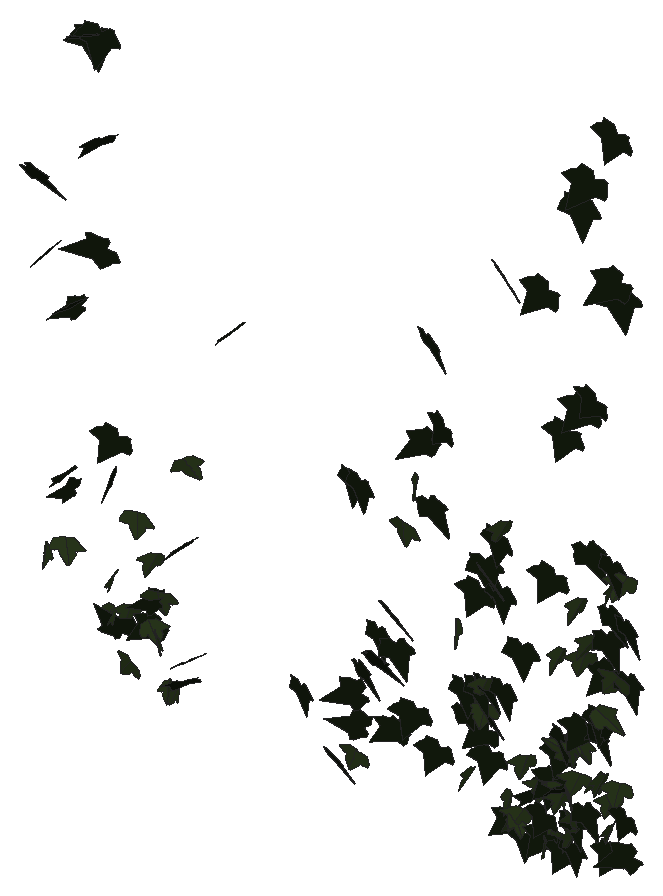
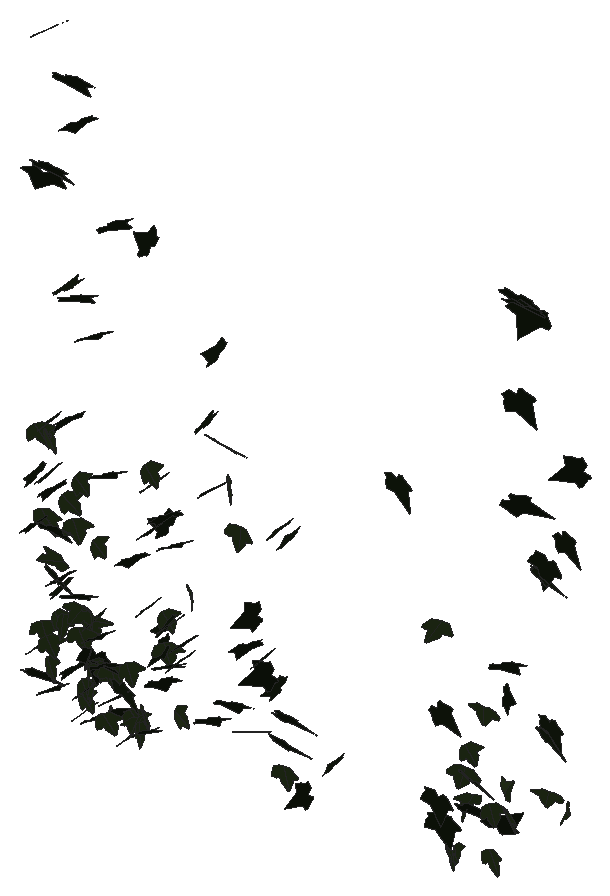
# SketchUp Ruby script. Lengths in inches.
U = 1.inch
M = Sketchup.active_model
def pt(a) = Geom::Point3d.new(a.map { |v| v * U })
def face(e, loops, mat)
  f = e.add_face(loops[0].map { |a| pt(a) })
  loops[1..].each { |l| e.add_face(l.map { |a| pt(a) }).erase! }
  f.material = f.back_material = mat if mat
  f
end
# faces: each face lists its corners as indices into pts; further lists are holes
def faces(e, pts, list, mat = nil) = list.each { |f| face(e, (f[0].is_a?(Array) ? f : [f]).map { |l| l.map { |i| pts[i] } }, mat) }
# xy, xz, yz: faces in a plane at the given z, y or x. An outline is a flat list of corners, or four numbers for a rectangle; further outlines are holes
def ring(l) = l.size == 4 ? [[l[0], l[1]], [l[2], l[1]], [l[2], l[3]], [l[0], l[3]]] : l.each_slice(2).to_a
def flat(e, list, mat, &to3) = list.each { |f| face(e, (f[0].is_a?(Array) ? f : [f]).map { |l| ring(l).map { |u, v| to3.(u, v) } }, mat) }
def xy(e, z, list, mat = nil) = flat(e, list, mat) { |x, y| [x, y, z] }
def xz(e, y, list, mat = nil) = flat(e, list, mat) { |x, z| [x, y, z] }
def yz(e, x, list, mat = nil) = flat(e, list, mat) { |y, z| [x, y, z] }
def lines(e, pts, list) = list.each { |a, b| e.add_line(pt(pts[a]), pt(pts[b])) }
# prism: a flat outline (further loops are holes) pulled along v
def prism(e, loops, v, mat = nil)
  f = face(e, loops, mat); d = Geom::Vector3d.new(v.map { |x| x * U })
  f.pushpull(f.normal.samedirection?(d) ? d.length : -d.length)
end
def box(e, o, s, mat = nil) = prism(e, [[o, [o[0] + s[0], o[1], o[2]], [o[0] + s[0], o[1] + s[1], o[2]], [o[0], o[1] + s[1], o[2]]]], [0, 0, s[2]], mat)
def at(x, y, z, deg = 0) = Geom::Transformation.translation(pt([x, y, z])) * Geom::Transformation.rotation(ORIGIN, Z_AXIS, deg.degrees)
def axes(o, x, y, z) = Geom::Transformation.new([*x, 0, *y, 0, *z, 0, *pt(o).to_a, 1])
def part(name) = M.definitions.add(name)
# library, detail: a bought-in or finely detailed component or shape, given as its bounding box
def library(name, o, s) = part(name).tap { |d| box(d.entities, o, s) }
def detail(e, o, s) = box(e.add_group.entities, o, s)
def put(e, d, t, mat = nil) = e.add_instance(d, t).tap { |i| i.material = mat if mat }
def group(e, t, mat = nil) = e.add_group.tap { |g| g.transformation = t; g.material = mat if mat }.entities
root = M.entities
M.materials.add("1026 AP 7946 SUNNY SIDE UP").color = [254, 231, 186]
M.materials.add("efeu1").color = [18, 25, 13]
M.materials.add("efeu2").color = [43, 57, 29]
c1 = part("ivyleaf_9")
p = [[1.54,2.16,1.25],[1.36,2.04,1.19],[-0.21,0.99,0.68],[-0.71,1.11,0.82],[-0.85,0.86,0.67],[-0.8,0.17,0.21],
  [-0.9,-0.01,0.1],[-0.67,-0.16,-0.02],[-0.08,-0.08,-0.05],[-0.03,-0.6,-0.4],[0.65,-0.88,-0.66],[0.83,-0.6,-0.49],
  [1.29,-0.42,-0.43],[1.8125,-0.07,-0.26],[1.21,0.44,0.15]]
faces(c1.entities,p,[[0,1,2,3,4,5,6,7,8,9,10,11,12,13,14]],"efeu1")
c2 = part("ivyleaf_10")
p = [[0,0.5,-0.03],[-0.0625,2.02,-0.43],[-0.19,2.01,-0.46],[-0.54,1.05,-0.29],[-0.52,0.625,-0.18],[-0.83,0.76,-0.28],
  [-1.16,0.64,-0.33],[-1.15,0.33,-0.24],[-0.77,-0.39,0.02],[-0.3,-0.51,0.16],[0.04,-0.48,0.23],[-0.02,2.01,-0.4375],
  [-0.06,2.01,-0.43],[0.04,-0.49,0.23],[0.67,-0.49,0.14],[1.38,0.36,-0.2],[1.375,0.51,-0.24],[0.81,0.65,-0.19],
  [0.62,0.59,-0.15],[0.6,1.09,-0.28],[0.5,1.23,-0.31]]
faces(c2.entities,p,[[0,1,2,3,4,5,6,7,8,9,10],[11,12,0,13,14,15,16,17,18,19,20]],"efeu2")
put(root,c1,axes([92.76,212.33,309.97],[0.61577,-0.10114,0.08621],[0.11486,-0.06042,-0.40182],[0.18865,0.36692,-0.03675]),"1026 AP 7946 SUNNY SIDE UP")
put(root,c1,axes([93.45,212.58,306.92],[-0.2298,0.32016,-0.13975],[0.08656,-0.1247,-0.37388],[-0.58325,-0.14465,-0.00043]),"1026 AP 7946 SUNNY SIDE UP")
put(root,c2,axes([93.38,212.5,295.07],[-0.02793,0.21923,-0.27285],[-0.01306,-0.2582,-0.23822],[-0.57422,-0.00479,0.01869]),"1026 AP 7946 SUNNY SIDE UP")
put(root,c1,axes([94.39,212.21,298.42],[-0.11098,0.34417,0.06318],[-0.03773,0.05125,-0.37411],[-0.59033,-0.06798,0.01203]),"1026 AP 7946 SUNNY SIDE UP")
put(root,c2,axes([94.16,212.53,295.5625],[0.52881,0.11571,0.0689],[0.11671,-0.00528,-0.35454],[-0.19063,0.31775,-0.02595]),"1026 AP 7946 SUNNY SIDE UP")
put(root,c1,axes([94.67,212.66,305.0625],[-0.51376,0.19612,-0.06721],[0.01225,-0.10575,-0.37708],[-0.3507,-0.291,0.08529]),"1026 AP 7946 SUNNY SIDE UP")
put(root,c1,axes([94.69,212.27,297.96],[-0.38076,0.27164,0.01445],[-0.03395,-0.00362,-0.37671],[-0.46018,-0.22449,0.01583]),"1026 AP 7946 SUNNY SIDE UP")
put(root,c1,axes([94.6,212.12,305.27],[0.14247,0.35425,0.11205],[0.00975,0.10134,-0.3879],[-0.6248,0.08236,0.0195]),"1026 AP 7946 SUNNY SIDE UP")
put(root,c1,axes([95.09,212.29,316.06],[0.47035,0.31068,0.05928],[-0.02815,0.08266,-0.43872],[-0.5338,0.26939,0.07537]),"1026 AP 7946 SUNNY SIDE UP")
put(root,c1,axes([95.8,212.66,307.74],[-0.10303,-0.08129,-0.39977],[-0.38932,-0.29335,0.10448],[-0.51672,0.23723,0.00098]),"1026 AP 7946 SUNNY SIDE UP")
put(root,c1,axes([95.82,212.41,312.1875],[-0.07673,0.3426,-0.20544],[-0.01788,-0.19862,-0.37118],[-0.67009,-0.03393,0.03343]),"1026 AP 7946 SUNNY SIDE UP")
put(root,c1,axes([95.49,212.48,316.25],[-0.40695,-0.24543,-0.24571],[0.43304,0.04505,-0.34098],[0.36556,-0.32658,0.13039]),"1026 AP 7946 SUNNY SIDE UP")
put(root,c1,axes([95.88,212.35,316.48],[-0.54501,-0.14123,-0.22991],[0.36523,0.03495,-0.37167],[0.2339,-0.38365,0.04465]),"1026 AP 7946 SUNNY SIDE UP")
put(root,c1,axes([96.36,212.66,300.47],[-0.43398,-0.25244,0.05353],[-0.03118,-0.05703,-0.38432],[0.43686,-0.25484,0.02575]),"1026 AP 7946 SUNNY SIDE UP")
put(root,c2,axes([96.3125,212.5,294.95],[-0.13702,-0.0091,-0.36236],[-0.03469,-0.34708,0.01037],[-0.57353,0.02317,0.08594]),"1026 AP 7946 SUNNY SIDE UP")
put(root,c1,axes([96.3125,212.52,299.07],[-0.18552,0.03168,-0.36972],[0.4272,-0.24251,-0.11233],[-0.40607,-0.2696,0.05073]),"1026 AP 7946 SUNNY SIDE UP")
put(root,c2,axes([96.43,212.23,293.77],[0.36982,-0.24987,-0.03818],[-0.05471,0.01486,-0.35436],[0.4242,0.21975,-0.01241]),"1026 AP 7946 SUNNY SIDE UP")
put(root,c1,axes([96.85,212.26,293.11],[0.19309,0.02805,0.35312],[-0.55423,0.06471,0.11568],[-0.08889,-0.3425,0.04579]),"1026 AP 7946 SUNNY SIDE UP")
put(root,c2,axes([97.13,212.41,291.84],[-0.44163,0.1062,0.2101],[-0.32935,0.03695,-0.29834],[-0.18291,-0.32294,0.0299]),"1026 AP 7946 SUNNY SIDE UP")
put(root,c2,axes([96.99,212.56,293.95],[-0.27729,-0.29083,0.06551],[0.01248,-0.07802,-0.35511],[0.50572,-0.15754,0.04469]),"1026 AP 7946 SUNNY SIDE UP")
put(root,c2,axes([97.54,212.21,297.9],[0.57977,0.00723,0.05775],[0.09081,0.01514,-0.36521],[-0.01612,0.34542,0.01963]),"1026 AP 7946 SUNNY SIDE UP")
put(root,c1,axes([98.17,212.6,293.65],[-0.544,-0.05543,0.0581],[-0.08436,-0.0344,-0.34762],[0.10224,-0.32332,0.02233]),"1026 AP 7946 SUNNY SIDE UP")
put(root,c2,axes([98,212.68,296.24],[-0.19952,-0.30194,0.13893],[-0.00662,-0.14065,-0.34565],[0.56052,-0.10914,0.04537]),"1026 AP 7946 SUNNY SIDE UP")
put(root,c1,axes([98.43,212.28,294.84],[-0.45298,0.21964,0.03461],[-0.0944,-0.02605,-0.36872],[-0.33608,-0.28872,0.05692]),"1026 AP 7946 SUNNY SIDE UP")
put(root,c2,axes([98.22,212.18,293.85],[0.28342,0.28049,0.09923],[0.04661,0.08707,-0.34757],[-0.49737,0.16799,0.02397]),"1026 AP 7946 SUNNY SIDE UP")
put(root,c2,axes([98.44,212.39,295.01],[-0.55179,-0.10051,-0.04825],[0.08139,-0.00722,-0.36366],[0.16735,-0.3279,0.01778]),"1026 AP 7946 SUNNY SIDE UP")
put(root,c2,axes([98.48,212.21,293.48],[-0.29828,0.28417,0.04966],[-0.08846,0.01768,-0.3555],[-0.47971,-0.17996,0.03468]),"1026 AP 7946 SUNNY SIDE UP")
put(root,c2,axes([98.71,212.51,291.54],[0.00491,-0.31439,0.09799],[0.17001,-0.09024,-0.32211],[0.53129,0.03178,0.10217]),"1026 AP 7946 SUNNY SIDE UP")
put(root,c2,axes([98.96,212.58,291.42],[0.3772,-0.23837,-0.04113],[-0.00122,0.04737,-0.34657],[0.40905,0.21995,0.03689]),"1026 AP 7946 SUNNY SIDE UP")
put(root,c1,axes([99.5,212.53,297.37],[-0.24023,0.28037,-0.20072],[0.05362,-0.20157,-0.3249],[-0.53561,-0.14593,0.0575]),"1026 AP 7946 SUNNY SIDE UP")
put(root,c1,axes([99.75,211.99,292.24],[0.1229,0.34201,-0.07529],[-0.10599,-0.06253,-0.37172],[-0.58476,0.08321,0.05155]),"1026 AP 7946 SUNNY SIDE UP")
put(root,c1,axes([99.99,211.99,293.14],[0.09011,0.35225,0.06284],[-0.05127,0.05895,-0.37835],[-0.6028,0.04764,0.04157]),"1026 AP 7946 SUNNY SIDE UP")
put(root,c2,axes([99.73,212.27,300.82],[-0.35864,-0.2511,-0.18487],[0.25136,0.09271,-0.34517],[0.4136,-0.27408,0.04947]),"1026 AP 7946 SUNNY SIDE UP")
put(root,c1,axes([101.59,212.46,306.54],[-0.14057,0.39503,-0.00121],[-0.01341,-0.00543,-0.41716],[-0.62102,-0.0893,0.00928]),"1026 AP 7946 SUNNY SIDE UP")
put(root,c1,axes([104.39,212.8,293.33],[0.08514,-0.33489,0.13186],[0.00493,-0.13092,-0.34982],[0.56478,0.05163,-0.01683]),"1026 AP 7946 SUNNY SIDE UP")
put(root,c1,axes([105.95,212.45,291.38],[0.52028,-0.1702,-0.03005],[-0.06115,-0.01416,-0.38214],[0.26429,0.33178,-0.02927]),"1026 AP 7946 SUNNY SIDE UP")
put(root,c1,axes([106.58,212.85,302.33],[0.03148,-0.34089,0.19903],[0.00021,-0.19538,-0.35278],[0.61761,0.01744,-0.01002]),"1026 AP 7946 SUNNY SIDE UP")
put(root,c1,axes([107.32,212.34,294.28],[-0.56788,0.06211,0.12333],[-0.19615,-0.02638,-0.37484],[-0.07932,-0.37945,0.04396]),"1026 AP 7946 SUNNY SIDE UP")
put(root,c2,axes([107.23,212.29,291.88],[-0.52801,0.04641,0.11954],[-0.19129,-0.04843,-0.34377],[-0.04332,-0.35188,0.06095]),"1026 AP 7946 SUNNY SIDE UP")
put(root,c1,axes([107.53,212.26,293.06],[-0.38427,0.1589,0.22422],[-0.34435,0.05207,-0.2934],[-0.24496,-0.32247,0.06071]),"1026 AP 7946 SUNNY SIDE UP")
put(root,c1,axes([107.15,212.64,302.49],[0.02786,-0.37071,0.13348],[0.00817,-0.13158,-0.38311],[0.61854,0.01843,-0.00095]),"1026 AP 7946 SUNNY SIDE UP")
put(root,c1,axes([107.41,212.29,295.43],[0.33607,-0.32348,0.0119],[-0.01669,-0.02304,-0.39893],[0.5088,0.2129,-0.02095]),"1026 AP 7946 SUNNY SIDE UP")
put(root,c1,axes([107.81,212.81,296.75],[0.06498,-0.36544,0.07076],[-0.0077,-0.07172,-0.37907],[0.58525,0.03963,-0.01285]),"1026 AP 7946 SUNNY SIDE UP")
put(root,c1,axes([107.82,212.41,295.88],[0.58312,-0.09763,0.07354],[0.09192,-0.05887,-0.3931],[0.16707,0.37314,-0.04039]),"1026 AP 7946 SUNNY SIDE UP")
put(root,c1,axes([108.78,212.71,293.22],[-0.47428,-0.14407,0.14753],[-0.06989,-0.2046,-0.30792],[0.31261,-0.26432,0.155]),"1026 AP 7946 SUNNY SIDE UP")
put(root,c1,axes([108.55,212.28,298.15],[0.53786,-0.20306,0.00164],[-0.02065,-0.02749,-0.40877],[0.31865,0.34097,-0.02926]),"1026 AP 7946 SUNNY SIDE UP")
put(root,c1,axes([108.94,212.36,296.77],[-0.03467,-0.37319,-0.13431],[0.01555,0.12789,-0.38437],[0.62029,-0.02406,0.00213]),"1026 AP 7946 SUNNY SIDE UP")
put(root,c2,axes([109.29,212.4,301.58],[-0.58905,0.10382,0.03928],[-0.07359,-0.02909,-0.39848],[-0.15722,-0.37537,0.03937]),"1026 AP 7946 SUNNY SIDE UP")
put(root,c1,axes([109.49,212.73,294.22],[-0.43258,-0.24305,-0.05714],[0.13844,-0.01956,-0.37091],[0.36623,-0.27969,0.07272]),"1026 AP 7946 SUNNY SIDE UP")
put(root,c2,axes([109.79,212.39,303.51],[0.27299,-0.35416,-0.05085],[0.04921,0.06751,-0.40162],[0.55968,0.16681,0.06012]),"1026 AP 7946 SUNNY SIDE UP")
put(root,c1,axes([110.26,212.58,305.25],[-0.62794,0.01764,-0.04299],[0.05227,-0.13862,-0.38795],[-0.04861,-0.37685,0.13819]),"1026 AP 7946 SUNNY SIDE UP")
put(root,c1,axes([110.05,212.73,309.19],[0.28418,-0.35183,0.13106],[0.05181,-0.12799,-0.40723],[0.58707,0.1816,-0.02751]),"1026 AP 7946 SUNNY SIDE UP")
put(root,c1,axes([110.58,212.69,293.1],[-0.34561,-0.2899,0.04054],[0.02481,-0.06291,-0.37156],[0.4597,-0.21455,0.05053]),"1026 AP 7946 SUNNY SIDE UP")
put(root,c1,axes([110.52,212.26,303.02],[0.14494,-0.37106,-0.10672],[0.03381,0.10916,-0.39043],[0.60394,0.08294,0.04747]),"1026 AP 7946 SUNNY SIDE UP")
put(root,c1,axes([110.7,212.81,305.83],[-0.1396,-0.2355,0.32488],[-0.04872,-0.31945,-0.25553],[0.61864,-0.0783,0.05319]),"1026 AP 7946 SUNNY SIDE UP")
put(root,c2,axes([111.375,212.71,298.25],[-0.29683,0.24921,-0.23039],[0.01618,-0.25376,-0.29986],[-0.52775,-0.14795,0.12039]),"1026 AP 7946 SUNNY SIDE UP")
put(root,c1,axes([111.76,212.68,295.98],[-0.01895,-0.37074,0.06366],[-0.00045,-0.06393,-0.38251],[0.59155,-0.01192,0.00175]),"1026 AP 7946 SUNNY SIDE UP")
put(root,c2,axes([112.07,212.57,292.76],[0.09882,-0.30776,0.18989],[0.03267,-0.18547,-0.32434],[0.56455,0.0646,-0.01447]),"1026 AP 7946 SUNNY SIDE UP")
put(root,c1,axes([111.87,212.46,295.23],[0.21872,-0.31701,-0.14947],[-0.05198,0.14158,-0.35491],[0.54455,0.14084,0.02616]),"1026 AP 7946 SUNNY SIDE UP")
put(root,c1,axes([112.37,212.72,300.01],[-0.28977,-0.3244,0.11851],[0.00763,-0.13495,-0.37877],[0.54213,-0.17149,0.06867]),"1026 AP 7946 SUNNY SIDE UP")
put(root,c2,axes([112.6875,212.61,295.4375],[-0.42174,-0.24526,0.08988],[0.01028,-0.13343,-0.36077],[0.40994,-0.24898,0.10151]),"1026 AP 7946 SUNNY SIDE UP")
put(root,c1,axes([112.75,212.65,294.61],[-0.39792,-0.22093,0.16301],[-0.07115,-0.18057,-0.3327],[0.4225,-0.23848,0.0975]),"1026 AP 7946 SUNNY SIDE UP")
put(root,c1,axes([112.52,212.39,296.49],[0.07628,-0.37578,-0.00629],[0.00136,0.00411,-0.39032],[0.59091,0.0485,0.00171]),"1026 AP 7946 SUNNY SIDE UP")
put(root,c1,axes([112.61,212.72,301.21],[-0.07166,-0.38594,-0.07628],[0.02447,0.0705,-0.39987],[0.61679,-0.04764,0.007]),"1026 AP 7946 SUNNY SIDE UP")
put(root,c2,axes([112.88,212.36,296.64],[-0.14948,-0.33316,0.15162],[0.0167,-0.1565,-0.35427],[0.57367,-0.08226,0.04982]),"1026 AP 7946 SUNNY SIDE UP")
put(root,c1,axes([112.57,212.65,296.49],[0.26184,-0.33798,0.03074],[0.00159,-0.03488,-0.38807],[0.53378,0.1659,-0.01392]),"1026 AP 7946 SUNNY SIDE UP")
put(root,c1,axes([112.52,212.72,300.82],[0.27578,-0.28479,0.21287],[0.14109,-0.18891,-0.34509],[0.53651,0.19606,-0.01867]),"1026 AP 7946 SUNNY SIDE UP")
put(root,c1,axes([112.72,212.53,295.49],[0.4477,-0.22274,-0.16021],[-0.21489,0.07514,-0.37122],[0.36786,0.31498,-0.02187]),"1026 AP 7946 SUNNY SIDE UP")
put(root,c1,axes([113.05,212.5,293.81],[-0.27158,-0.32542,-0.00198],[0.00749,-0.00244,-0.37951],[0.51164,-0.1727,0.0045]),"1026 AP 7946 SUNNY SIDE UP")
put(root,c1,axes([113.22,212.7,302.38],[-0.07425,-0.36005,0.16836],[0.00465,-0.16696,-0.37436],[0.62305,-0.04166,0.02286]),"1026 AP 7946 SUNNY SIDE UP")
put(root,c2,axes([113.45,212.69,302.93],[-0.08907,-0.37004,0.14562],[-0.00175,-0.14476,-0.38599],[0.62405,-0.05322,0.01971]),"1026 AP 7946 SUNNY SIDE UP")
put(root,c1,axes([113.33,212.73,300.34],[-0.02505,-0.38348,0.0777],[-0.00979,-0.0774,-0.39584],[0.61513,-0.01685,-0.00313]),"1026 AP 7946 SUNNY SIDE UP")
put(root,c1,axes([113.28,212.84,312.76],[0.19804,-0.27752,0.30493],[0.1609,-0.27988,-0.31516],[0.61924,0.16148,-0.01563]),"1026 AP 7946 SUNNY SIDE UP")
put(root,c2,axes([113.67,212.68,292.3],[0.33778,-0.28088,0.05386],[0.06429,-0.03652,-0.36435],[0.44508,0.21844,0.01176]),"1026 AP 7946 SUNNY SIDE UP")
put(root,c1,axes([113.875,212.74,291.37],[-0.35189,-0.19692,0.20702],[-0.13198,-0.19978,-0.2975],[0.42358,-0.22584,0.07929]),"1026 AP 7946 SUNNY SIDE UP")
put(root,c1,axes([113.6875,212.375,296.75],[0.05324,-0.37034,0.06676],[-0.00059,-0.06721,-0.38345],[0.59174,0.03325,-0.00639]),"1026 AP 7946 SUNNY SIDE UP")
put(root,c2,axes([113.95,212.56,291.51],[0.00925,-0.35273,-0.08524],[0.03487,0.08095,-0.36219],[0.56791,0.00077,0.02363]),"1026 AP 7946 SUNNY SIDE UP")
put(root,c2,axes([114.33,212.52,291.92],[-0.31828,-0.25071,0.17213],[-0.06358,-0.17853,-0.32472],[0.47071,-0.19364,0.07253]),"1026 AP 7946 SUNNY SIDE UP")
put(root,c2,axes([114.18,212.48,291.75],[0.17444,0.34119,0.01481],[0.03131,0.00659,-0.36916],[-0.53593,0.11144,-0.01675]),"1026 AP 7946 SUNNY SIDE UP")
put(root,c2,axes([114.4,212.7,293.99],[-0.23901,-0.32785,0.07921],[0.02709,-0.09382,-0.36868],[0.52948,-0.14319,0.05462]),"1026 AP 7946 SUNNY SIDE UP")
put(root,c1,axes([114.36,212.71,290.99],[-0.0436,-0.33417,0.11668],[0.01322,-0.1161,-0.34568],[0.55562,-0.02346,0.01738]),"1026 AP 7946 SUNNY SIDE UP")
put(root,c1,axes([114.5,212.41,298.6],[-0.11185,-0.37995,-0.02259],[0.00906,0.01904,-0.3981],[0.59817,-0.07133,0.00181]),"1026 AP 7946 SUNNY SIDE UP")
put(root,c1,axes([114.98,212.41,292.89],[-0.2038,0.33206,0.06533],[-0.10594,0.03915,-0.36367],[-0.52034,-0.13803,0.04846]),"1026 AP 7946 SUNNY SIDE UP")
put(root,c1,axes([115.3,212.76,312.88],[-0.36738,-0.30189,0.19767],[-0.15253,-0.16924,-0.39348],[0.54289,-0.25184,0.02321]),"1026 AP 7946 SUNNY SIDE UP")
put(root,c2,axes([115.4,212.47,293.44],[-0.46875,-0.19675,0.07023],[-0.06186,-0.06566,-0.36682],[0.32211,-0.29893,0.03176]),"1026 AP 7946 SUNNY SIDE UP")
put(root,c2,axes([115.5,212.7,291.43],[-0.31805,-0.25002,0.16116],[-0.074,-0.1616,-0.32674],[0.45901,-0.19929,0.059]),"1026 AP 7946 SUNNY SIDE UP")
put(root,c1,axes([115.4,212.5625,292.2],[-0.20451,-0.29488,0.17573],[-0.03763,-0.176,-0.33004],[0.53567,-0.12494,0.04391]),"1026 AP 7946 SUNNY SIDE UP")
put(root,c1,axes([115.55,212.42,291.53],[-0.32331,-0.26693,0.1284],[-0.08921,-0.11514,-0.34693],[0.45559,-0.21198,0.02319]),"1026 AP 7946 SUNNY SIDE UP")
put(root,c1,axes([115.74,212.75,293.64],[-0.40872,-0.22551,0.12154],[-0.07799,-0.12234,-0.3504],[0.39347,-0.2585,0.0568]),"1026 AP 7946 SUNNY SIDE UP")
put(root,c2,axes([115.7,212.1,291.36],[0.22946,-0.30539,-0.11619],[0.02244,0.12764,-0.34154],[0.51047,0.13166,0.06724]),"1026 AP 7946 SUNNY SIDE UP")
put(root,c2,axes([115.63,212.46,293.45],[-0.46856,-0.1327,-0.17327],[0.27078,0.02089,-0.33267],[0.19883,-0.34117,0.04473]),"1026 AP 7946 SUNNY SIDE UP")
put(root,c1,axes([115.77,212.5625,301.82],[-0.35199,-0.30882,0.10792],[0.00094,-0.12951,-0.3863],[0.51367,-0.21138,0.07466]),"1026 AP 7946 SUNNY SIDE UP")
put(root,c1,axes([115.71,212.65,293.63],[-0.43445,-0.19272,-0.1517],[0.29173,-0.02651,-0.32547],[0.244,-0.31145,0.11903]),"1026 AP 7946 SUNNY SIDE UP")
put(root,c2,axes([115.97,212.66,298.78],[-0.02909,-0.32138,0.21826],[0.07551,-0.21419,-0.32883],[0.60214,0.01134,0.05178]),"1026 AP 7946 SUNNY SIDE UP")
put(root,c1,axes([115.95,212.77,294.83],[-0.19694,-0.33442,0.105],[-0.00241,-0.10974,-0.3667],[0.5506,-0.1201,0.03595]),"1026 AP 7946 SUNNY SIDE UP")
put(root,c2,axes([116.23,212.42,293.37],[-0.1578,-0.33565,0.11967],[0.03324,-0.12808,-0.35735],[0.55849,-0.08721,0.05508]),"1026 AP 7946 SUNNY SIDE UP")
put(root,c1,axes([116.04,212.74,295.48],[0.04424,-0.34351,0.14383],[-0.00079,-0.14201,-0.35571],[0.5842,0.02582,-0.01137]),"1026 AP 7946 SUNNY SIDE UP")
put(root,c1,axes([116.34,212.24,293.67],[0.15539,0.34604,-0.05455],[-0.01018,-0.05525,-0.37096],[-0.55083,0.09864,-0.00853]),"1026 AP 7946 SUNNY SIDE UP")
put(root,c2,axes([116.64,212.42,295.14],[0.18628,0.09215,0.36401],[-0.52394,-0.12334,0.14773],[0.23292,-0.35114,0.04119]),"1026 AP 7946 SUNNY SIDE UP")
put(root,c1,axes([116.24,212.6,291.1],[-0.24012,-0.29566,0.14021],[-0.02875,-0.14414,-0.34036],[0.5121,-0.14673,0.04664]),"1026 AP 7946 SUNNY SIDE UP")
put(root,c1,axes([116.32,212.67,307.67],[-0.29672,-0.35246,0.11772],[0.00962,-0.13337,-0.40706],[0.58351,-0.17703,0.06657]),"1026 AP 7946 SUNNY SIDE UP")
put(root,c2,axes([116.37,212.6,292.49],[-0.37598,0.26177,-0.09683],[0.06818,-0.08932,-0.36469],[-0.4328,-0.24148,0.02666]),"1026 AP 7946 SUNNY SIDE UP")
put(root,c2,axes([116.57,212.66,292.49],[-0.09108,-0.35324,0.05346],[-0.00381,-0.05421,-0.36902],[0.56185,-0.05763,0.00616]),"1026 AP 7946 SUNNY SIDE UP")
put(root,c2,axes([116.54,212.46,295.48],[-0.41039,0.23368,-0.12473],[0.05817,-0.13806,-0.35361],[-0.4107,-0.25306,0.07455]),"1026 AP 7946 SUNNY SIDE UP")
put(root,c2,axes([116.66,212.54,291.91],[-0.0203,-0.34138,0.13566],[-0.00232,-0.13366,-0.35271],[0.57645,-0.01256,0.00336]),"1026 AP 7946 SUNNY SIDE UP")
put(root,c1,axes([116.43,212.72,292.35],[0.0802,-0.35411,-0.00731],[-0.0062,0.00457,-0.36853],[0.55683,0.05105,-0.00305]),"1026 AP 7946 SUNNY SIDE UP")
put(root,c2,axes([116.64,212.26,293.6875],[-0.25675,0.3249,0.01909],[-0.04582,0.00399,-0.37374],[-0.50948,-0.16409,0.02399]),"1026 AP 7946 SUNNY SIDE UP")
put(root,c1,axes([116.53,212.6875,291.35],[0.01505,-0.35415,0.08088],[-0.00366,-0.0806,-0.36542],[0.57107,0.00882,-0.00448]),"1026 AP 7946 SUNNY SIDE UP")
put(root,c2,axes([116.94,212.53,301.15],[-0.06035,-0.33965,0.20221],[0.03356,-0.20066,-0.35114],[0.61745,-0.02229,0.03885]),"1026 AP 7946 SUNNY SIDE UP")
put(root,c2,axes([116.83,212.58,295.6],[-0.54565,0.05111,-0.13402],[0.19524,-0.04883,-0.36045],[-0.10184,-0.36747,0.02703]),"1026 AP 7946 SUNNY SIDE UP")
put(root,c1,axes([116.8,212.8,316.85],[-0.1349,-0.43104,-0.02127],[0.00637,0.01775,-0.45266],[0.67834,-0.08588,0.00002]),"1026 AP 7946 SUNNY SIDE UP")
put(root,c2,axes([117.1,212.27,294.4],[-0.42116,-0.2244,0.11253],[-0.07185,-0.11528,-0.35595],[0.3867,-0.26583,0.05642]),"1026 AP 7946 SUNNY SIDE UP")
put(root,c1,axes([117.05,212.71,296.21],[-0.42597,-0.25766,0.06116],[0.04634,-0.11584,-0.37096],[0.4137,-0.25233,0.10453]),"1026 AP 7946 SUNNY SIDE UP")
put(root,c2,axes([117.2,212.47,299.16],[-0.34272,-0.31012,0.08848],[-0.01598,-0.09915,-0.38801],[0.50649,-0.21297,0.04763]),"1026 AP 7946 SUNNY SIDE UP")
put(root,c1,axes([117.26,212.56,309],[-0.4687,-0.27156,0.11817],[-0.04788,-0.13602,-0.40857],[0.462,-0.28959,0.07754]),"1026 AP 7946 SUNNY SIDE UP")
put(root,c1,axes([117.13,212.55,293.04],[0.07559,-0.34452,-0.11468],[-0.0107,0.10944,-0.35762],[0.56825,0.04789,0.00852]),"1026 AP 7946 SUNNY SIDE UP")
put(root,c1,axes([117.68,212.33,318.29],[-0.65457,-0.15096,-0.04433],[0.08013,-0.01718,-0.45499],[0.23306,-0.41807,0.03193]),"1026 AP 7946 SUNNY SIDE UP")
put(root,c2,axes([117.66,212.34,300],[-0.13058,-0.31474,0.22176],[-0.06212,-0.21386,-0.3363],[0.59795,-0.09095,0.01349]),"1026 AP 7946 SUNNY SIDE UP")
put(root,c1,axes([117.53,212.68,309.31],[-0.27125,-0.25388,0.29507],[-0.01589,-0.31249,-0.29199],[0.60332,-0.12237,0.12498]),"1026 AP 7946 SUNNY SIDE UP")
put(root,c1,axes([117.49,212.3,303.61],[0.09911,-0.36621,-0.15781],[0.01698,0.15454,-0.38029],[0.62269,0.05407,0.03549]),"1026 AP 7946 SUNNY SIDE UP")
put(root,c1,axes([117.66,212.8,296.8],[-0.08277,-0.36328,0.07771],[-0.01325,-0.07708,-0.3786],[0.58392,-0.05324,0.00242]),"1026 AP 7946 SUNNY SIDE UP")
put(root,c1,axes([117.66,212.58,296.3],[0.20526,-0.35185,0.01645],[-0.01118,-0.02178,-0.38647],[0.55386,0.12996,-0.0139]),"1026 AP 7946 SUNNY SIDE UP")
put(root,c2,axes([117.95,212.19,294.64],[-0.06954,-0.33884,-0.14525],[0.07341,0.13373,-0.35017],[0.57123,-0.05843,0.02732]),"1026 AP 7946 SUNNY SIDE UP")
put(root,c1,axes([118.28,212.56,296.77],[-0.47996,0.20953,-0.05897],[0.0453,-0.06086,-0.38021],[-0.33902,-0.30477,0.03268]),"1026 AP 7946 SUNNY SIDE UP")
put(root,c1,axes([118.22,212.72,298.79],[-0.57755,-0.10295,-0.03467],[0.07642,-0.05258,-0.3878],[0.15188,-0.36502,0.06329]),"1026 AP 7946 SUNNY SIDE UP")
put(root,c2,axes([118.13,212.3,294.73],[-0.01659,-0.35742,0.0947],[0.00916,-0.09414,-0.36882],[0.58103,-0.00872,0.00852]),"1026 AP 7946 SUNNY SIDE UP")
put(root,c2,axes([118.3,212.67,293.81],[-0.24355,-0.31641,0.12205],[0.00355,-0.13322,-0.35886],[0.53224,-0.1439,0.05824]),"1026 AP 7946 SUNNY SIDE UP")
put(root,c1,axes([118.5625,212.6875,314.37],[-0.67911,-0.05855,0.00937],[-0.00254,-0.05768,-0.44549],[0.09322,-0.42813,0.05615]),"1026 AP 7946 SUNNY SIDE UP")
put(root,c2,axes([118.35,212.52,292.79],[0.0469,-0.36637,-0.00906],[0.00039,0.00675,-0.37864],[0.57618,0.02982,0.00099]),"1026 AP 7946 SUNNY SIDE UP")
put(root,c1,axes([118.27,212.68,291.7],[-0.24443,-0.29476,0.13279],[-0.0267,-0.13727,-0.34087],[0.50621,-0.14957,0.04614]),"1026 AP 7946 SUNNY SIDE UP")
put(root,c1,axes([118.15,212.66,301.18],[0.23088,-0.36135,-0.06541],[-0.0312,0.05826,-0.40146],[0.5755,0.14812,0.00448]),"1026 AP 7946 SUNNY SIDE UP")
put(root,c1,axes([118.28,212.38,300.33],[0.05685,-0.37954,-0.09554],[-0.02453,0.08949,-0.39218],[0.61305,0.03878,-0.00683]),"1026 AP 7946 SUNNY SIDE UP")
put(root,c2,axes([118.04,212.34,297.22],[0.28058,0.07224,0.35255],[0.53758,0.04283,-0.19295],[-0.11298,0.38319,-0.04255]),"1026 AP 7946 SUNNY SIDE UP")
put(root,c2,axes([118.59,212.66,294.35],[-0.41864,-0.248,0.08864],[0.02054,-0.13677,-0.35939],[0.41299,-0.24459,0.10773]),"1026 AP 7946 SUNNY SIDE UP")
put(root,c1,axes([118.45,212.6875,320.22],[-0.24194,-0.37692,0.20004],[-0.00911,-0.20691,-0.41514],[0.66818,-0.1393,0.06677]),"1026 AP 7946 SUNNY SIDE UP")
put(root,c2,axes([118.84,212.22,298.89],[-0.51537,0.0078,0.2097],[-0.31605,-0.07449,-0.33099],[0.05157,-0.37854,0.06715]),"1026 AP 7946 SUNNY SIDE UP")
put(root,c2,axes([118.57,212.36,302.52],[0.14142,-0.37588,0.09899],[0.03311,-0.09596,-0.39872],[0.60999,0.09236,-0.00131]),"1026 AP 7946 SUNNY SIDE UP")
put(root,c1,axes([118.41,212.57,303.16],[0.04532,-0.38616,0.10386],[0.01272,-0.1027,-0.39953],[0.62831,0.02993,0.0006]),"1026 AP 7946 SUNNY SIDE UP")
put(root,c1,axes([118.58,212.62,313.96],[-0.39914,-0.21408,-0.29269],[0.3817,0.14887,-0.33957],[0.40681,-0.34972,0.03144]),"1026 AP 7946 SUNNY SIDE UP")
put(root,c2,axes([118.93,212.54,302.73],[-0.35181,-0.27479,0.19112],[-0.03231,-0.21365,-0.34985],[0.52171,-0.19853,0.10721]),"1026 AP 7946 SUNNY SIDE UP")
put(root,c1,axes([118.88,212.65,293.29],[-0.11849,-0.29541,0.1993],[-0.01103,-0.19823,-0.3131],[0.55659,-0.06682,0.03623]),"1026 AP 7946 SUNNY SIDE UP")
put(root,c1,axes([119.35,212.39,291.98],[-0.53541,-0.0312,0.13142],[-0.18888,-0.07052,-0.34799],[0.08415,-0.35678,0.05511]),"1026 AP 7946 SUNNY SIDE UP")
put(root,c1,axes([118.81,212.73,300.88],[0.22268,-0.36167,0.06668],[-0.00093,-0.07179,-0.39964],[0.57831,0.13915,-0.02632]),"1026 AP 7946 SUNNY SIDE UP")
put(root,c1,axes([118.9,212.75,298.73],[0.05575,-0.38041,-0.03034],[-0.01625,0.02644,-0.39336],[0.59948,0.03609,-0.00784]),"1026 AP 7946 SUNNY SIDE UP")
